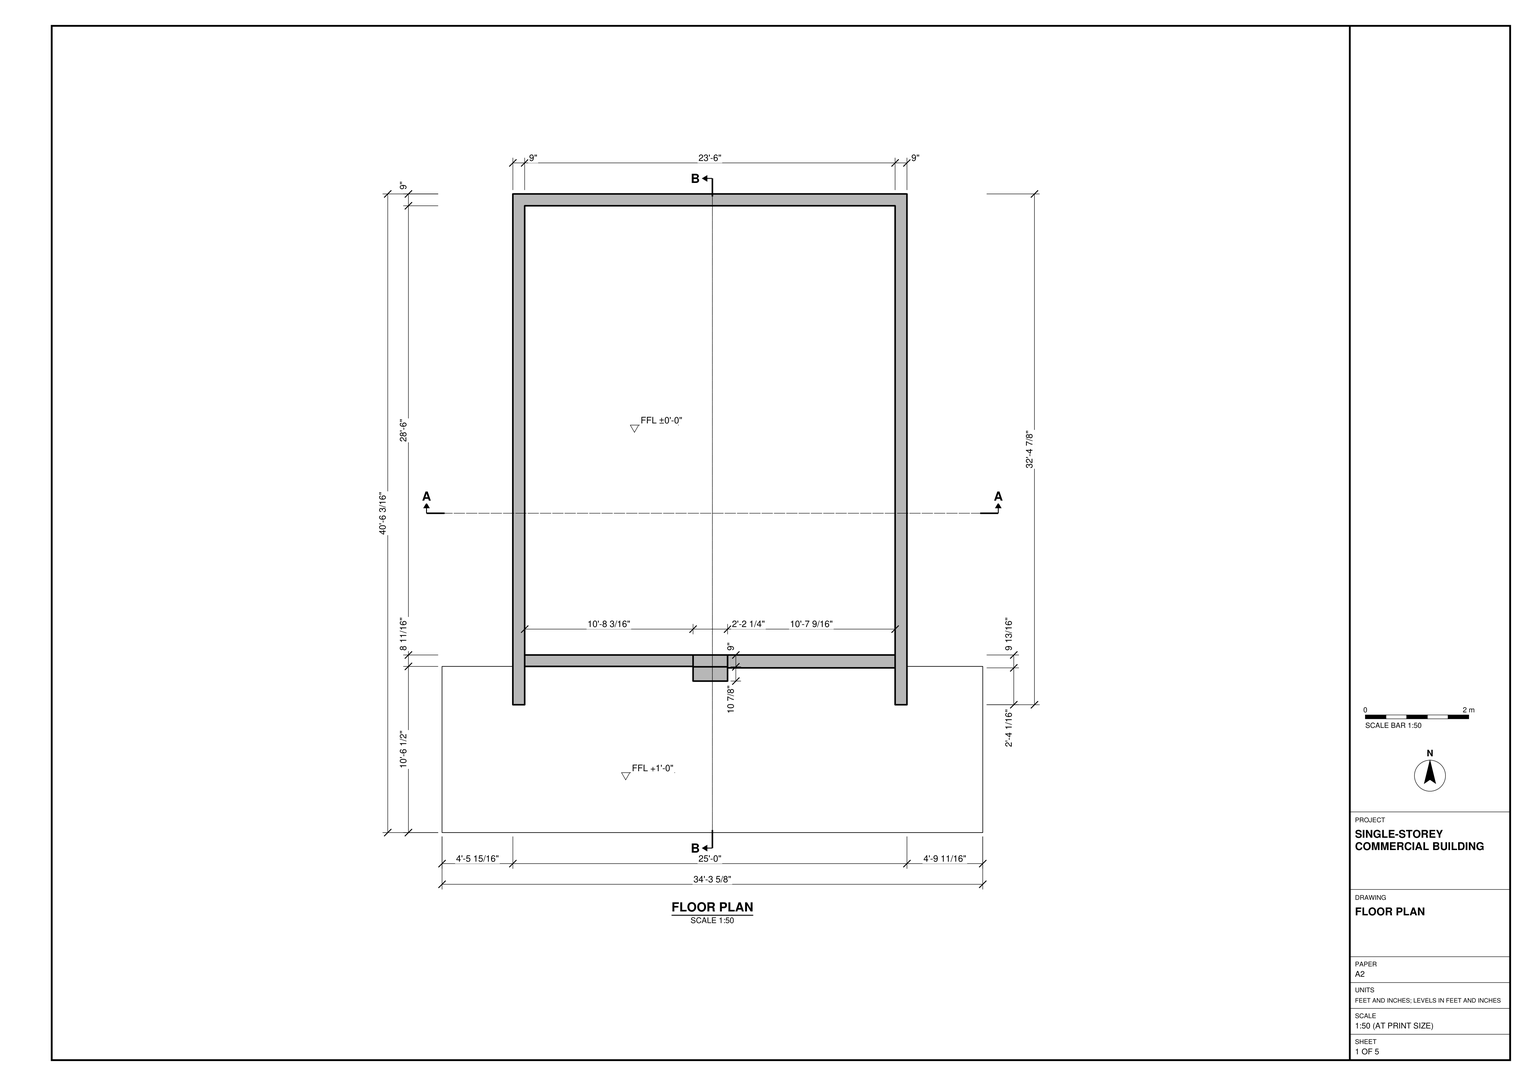
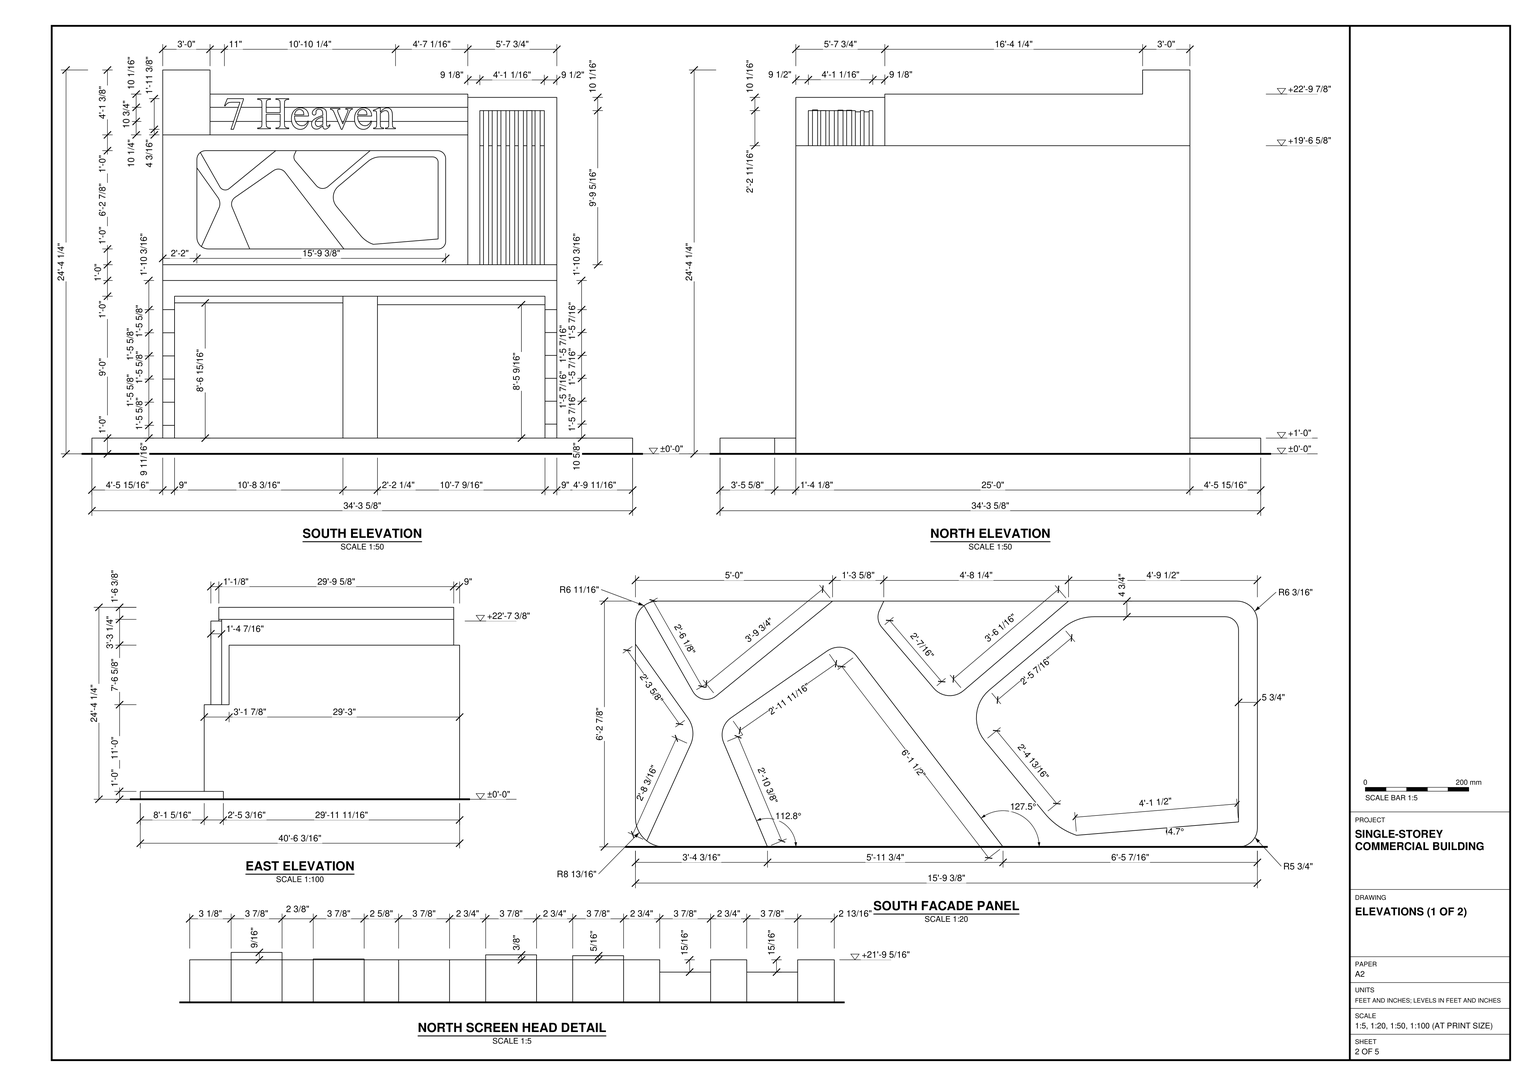
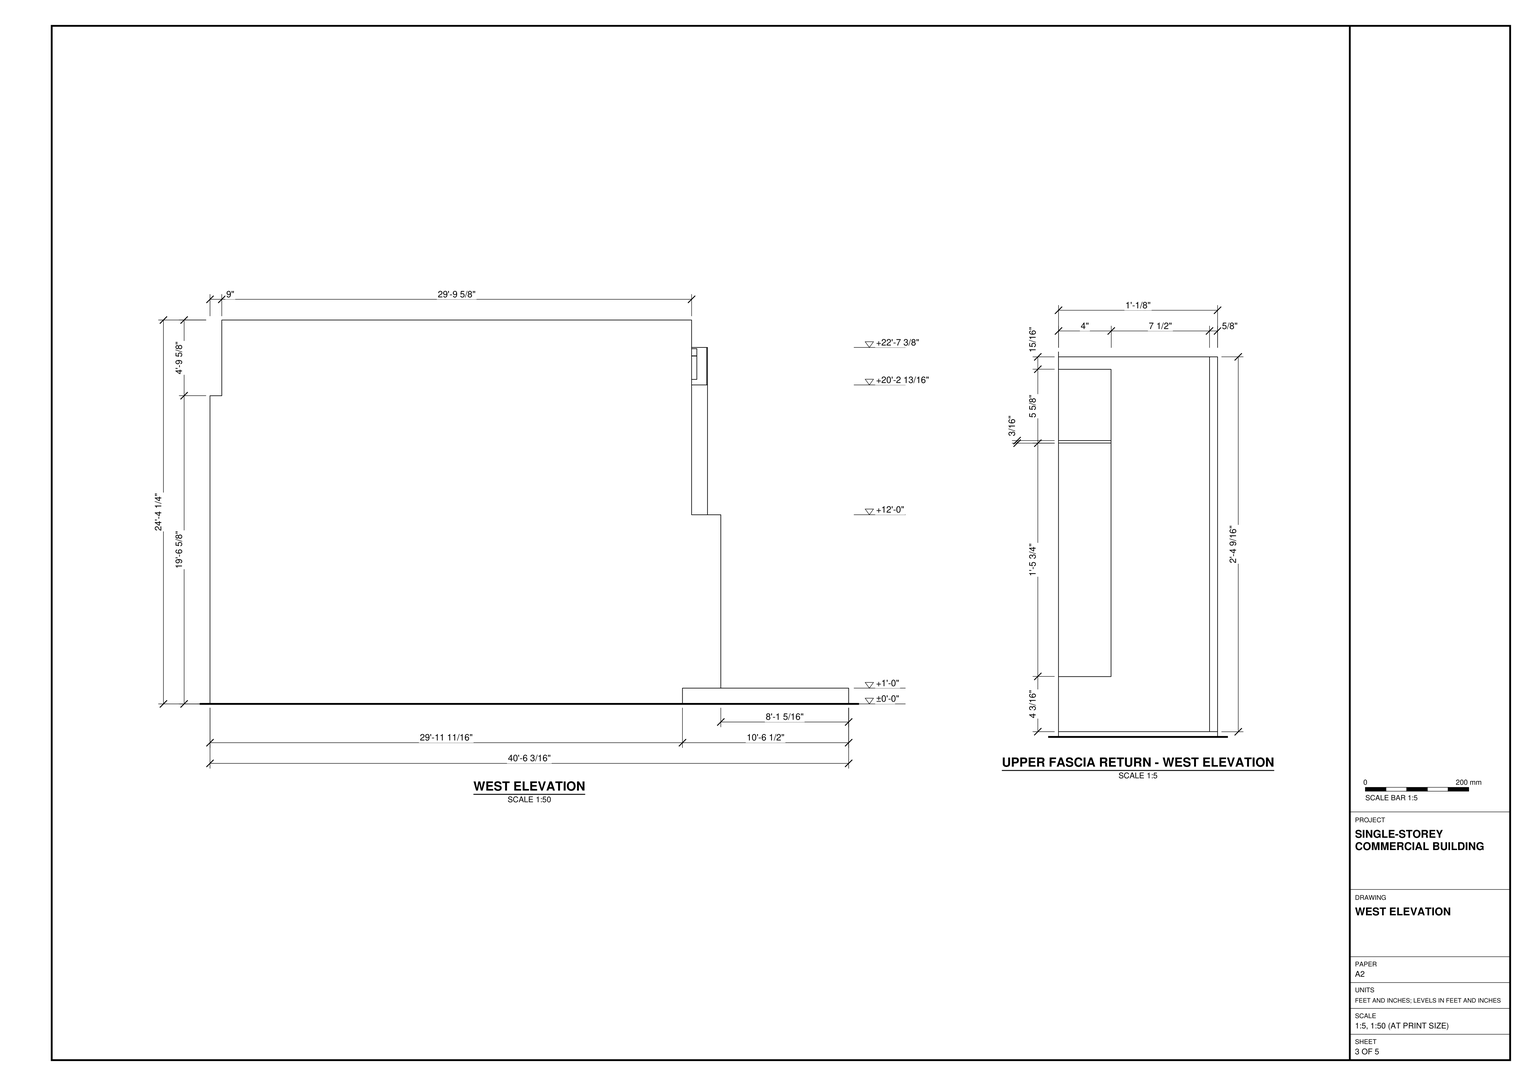
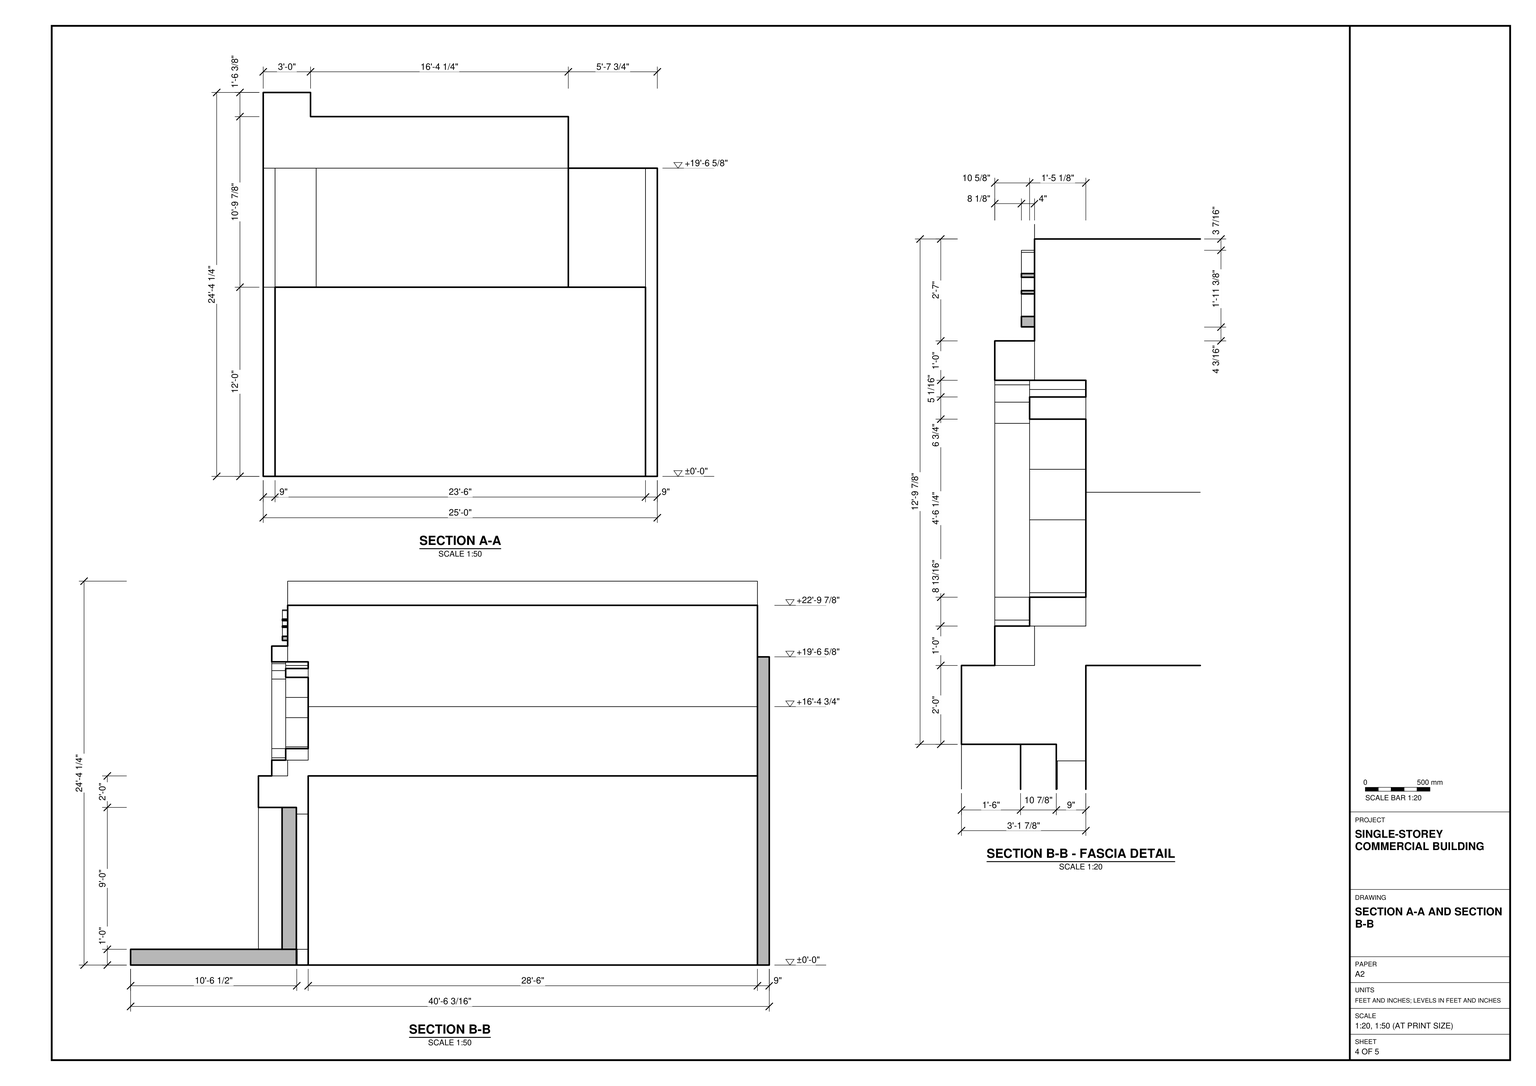
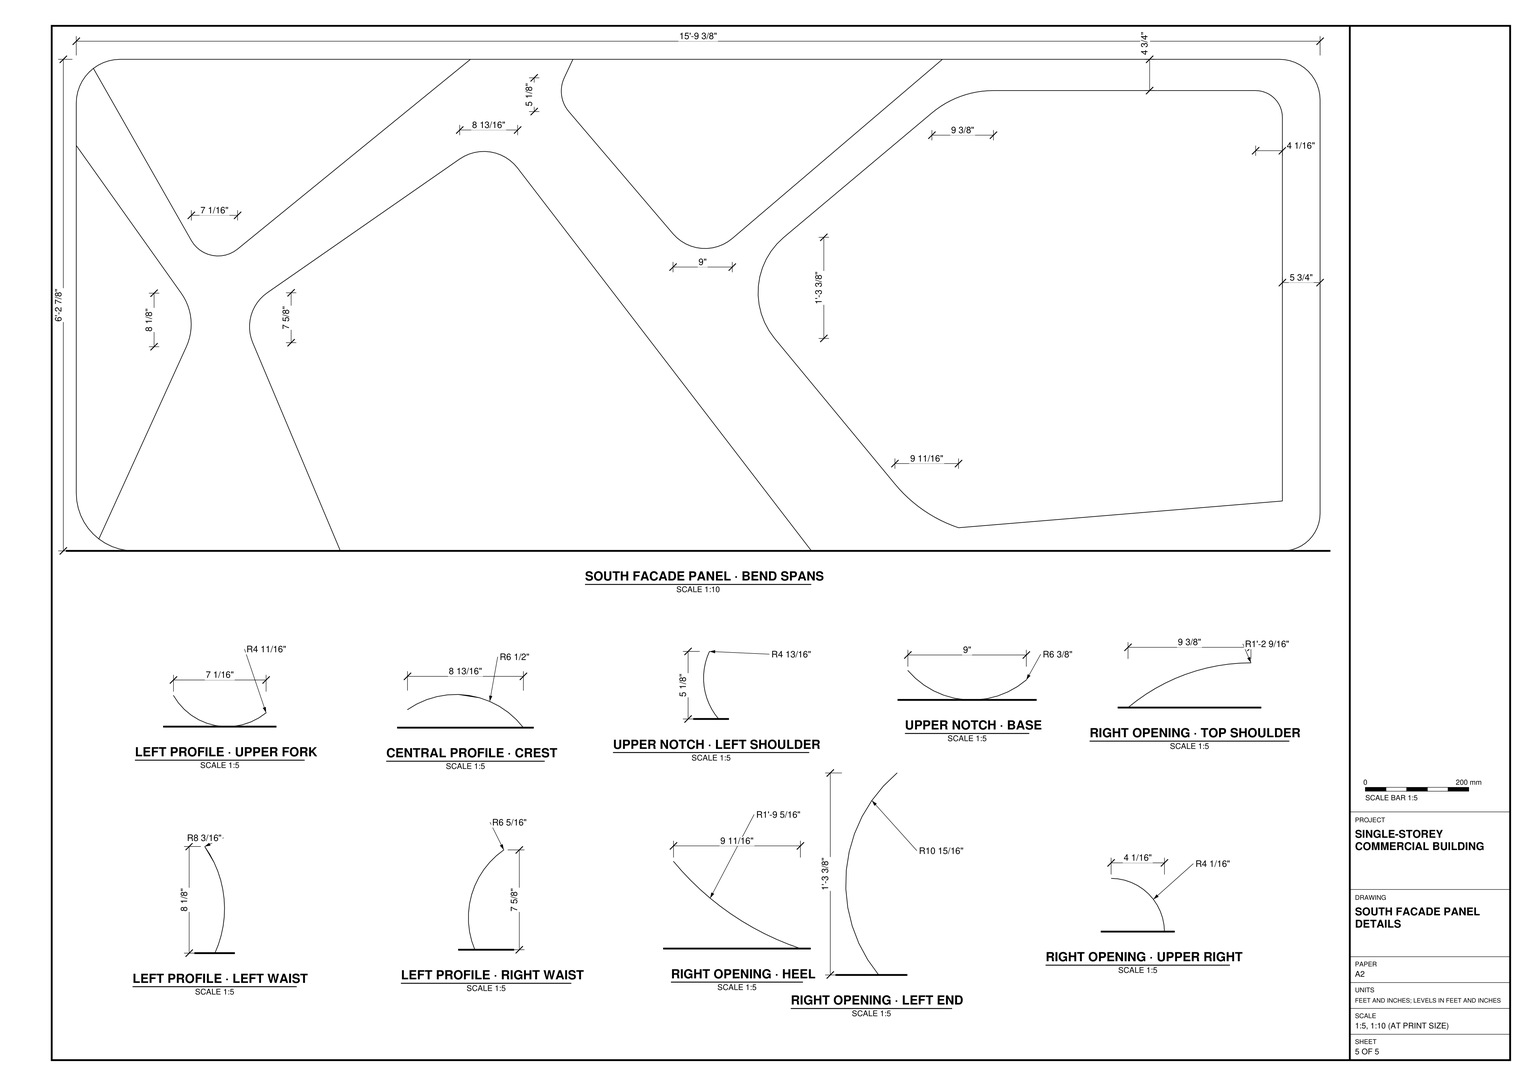
Use task_files/diagram_01.pdf to build the single-storey commercial building in SketchUp. Work in feet and inches. Set the ground-floor datum to ±0'-0". The complete model, including the projecting front platform, measures 34'-3 5/8" east to west, 40'-6 3/16" north to south and 24'-4 1/4" high.

Lay out the rectangular interior using the clear dimensions on the floor plan and the 9" side and rear walls. Extend the side walls past the storefront as drawn. Place the front platform at +1'-0" and follow the plan offsets on each side rather than centring it on the building. Form the two wide storefront bays on either side of the central pier, with a continuous horizontal band above them.

Use the south elevation and its enlarged panel detail to lay out the upper facade. Reproduce the rounded panel outline and branching diagonal pattern, the sign lettering on the horizontal fascia above it, and the narrow vertical screen to its right. Follow the side and rear elevations for the roof, stepped parapet heights and fascia returns.

Keep the walls, slabs, roof and distinct facade elements in separate groups or components, and use components for repeated parts such as screen slats. Any decor or loose items shown may be represented by suitable library components. Save one SketchUp model as output_files/single_storey_commercial_building_with_storefront.skp.

# SketchUp Ruby script. Lengths in inches.
U = 1.inch
M = Sketchup.active_model
def pt(a) = Geom::Point3d.new(a.map { |v| v * U })
def face(e, loops, mat)
  f = e.add_face(loops[0].map { |a| pt(a) })
  loops[1..].each { |l| e.add_face(l.map { |a| pt(a) }).erase! }
  f.material = f.back_material = mat if mat
  f
end
# faces: each face lists its corners as indices into pts; further lists are holes
def faces(e, pts, list, mat = nil) = list.each { |f| face(e, (f[0].is_a?(Array) ? f : [f]).map { |l| l.map { |i| pts[i] } }, mat) }
# xy, xz, yz: faces in a plane at the given z, y or x. An outline is a flat list of corners, or four numbers for a rectangle; further outlines are holes
def ring(l) = l.size == 4 ? [[l[0], l[1]], [l[2], l[1]], [l[2], l[3]], [l[0], l[3]]] : l.each_slice(2).to_a
def flat(e, list, mat, &to3) = list.each { |f| face(e, (f[0].is_a?(Array) ? f : [f]).map { |l| ring(l).map { |u, v| to3.(u, v) } }, mat) }
def xy(e, z, list, mat = nil) = flat(e, list, mat) { |x, y| [x, y, z] }
def xz(e, y, list, mat = nil) = flat(e, list, mat) { |x, z| [x, y, z] }
def yz(e, x, list, mat = nil) = flat(e, list, mat) { |y, z| [x, y, z] }
def lines(e, pts, list) = list.each { |a, b| e.add_line(pt(pts[a]), pt(pts[b])) }
# prism: a flat outline (further loops are holes) pulled along v
def prism(e, loops, v, mat = nil)
  f = face(e, loops, mat); d = Geom::Vector3d.new(v.map { |x| x * U })
  f.pushpull(f.normal.samedirection?(d) ? d.length : -d.length)
end
def box(e, o, s, mat = nil) = prism(e, [[o, [o[0] + s[0], o[1], o[2]], [o[0] + s[0], o[1] + s[1], o[2]], [o[0], o[1] + s[1], o[2]]]], [0, 0, s[2]], mat)
def at(x, y, z, deg = 0) = Geom::Transformation.translation(pt([x, y, z])) * Geom::Transformation.rotation(ORIGIN, Z_AXIS, deg.degrees)
def axes(o, x, y, z) = Geom::Transformation.new([*x, 0, *y, 0, *z, 0, *pt(o).to_a, 1])
def part(name) = M.definitions.add(name)
# library, detail: a bought-in or finely detailed component or shape, given as its bounding box
def library(name, o, s) = part(name).tap { |d| box(d.entities, o, s) }
def detail(e, o, s) = box(e.add_group.entities, o, s)
def put(e, d, t, mat = nil) = e.add_instance(d, t).tap { |i| i.material = mat if mat }
def group(e, t, mat = nil) = e.add_group.tap { |g| g.transformation = t; g.material = mat if mat }.entities
root = M.entities
M.materials.add("[Color B02]").color = [255, 178, 153]
M.materials.add("[Color B03]").color = [255, 140, 101]
M.materials.add("[Color M05]").color = [114, 114, 114]
M.materials.add("[Color M06]").color = [86, 86, 86]
M.materials.add("[Translucent Glass Gray]").color = [128, 128, 128]
M.materials["[Translucent Glass Gray]"].alpha = 0.5
M.materials.add("[Window Covering 02]").color = [199, 178, 115]
c1 = library("7 Heaven\#1",[1.28,0,0],[130.23,23.39,4])
xy(root,0,[[[53.91,126.2,353.91,486.2],[62.91,135.2,344.91,477.2]],[62.91,135.2,344.91,477.2]])
xy(root,12,[[53.91,97.32,62.91,126.2],[344.91,97.32,353.91,126.2],[191.1,115.32,217.37,126.2],[217.37,125.38,344.91,126.2],[62.91,126.2,191.1,126.51],
  [217.37,126.2,344.91,135.2],[62.91,126.51,191.1,135.2]])
xy(root,113.56,[[217.37,125.38,344.91,126.2],[217.37,126.2,344.91,135.2]])
xy(root,114.95,[[62.91,126.2,191.1,126.51],[62.91,126.51,191.1,135.2]])
xy(root,120,[[191.1,115.32,217.37,126.2]])
xy(root,120,[[62.91,97.32,191.1,126.2],[191.1,97.32,217.37,115.32],[217.37,97.32,344.91,126.2]],"[Color B03]")
xy(root,144,[[344.38,107.46,353.91,123.92],[298.1,108.67,301.98,123.92],[304.73,108.67,308.6,123.92],[311.35,108.67,315.23,123.92],[317.98,108.67,321.85,123.92],
  [324.6,108.67,328.48,123.92],[62.91,135.2,286.16,477.2],[286.16,135.2,344.91,477.2]])
xy(root,144,[[[53.91,97.32,353.91,97.32,353.91,107.46,344.38,107.46,344.38,123.92,353.91,123.92,353.91,135.2,286.16,135.2,286.16,123.92,295.3125,123.92,295.3125,107.46,53.91,107.46],[337.35,108.67,341.23,123.92],[331.1,108.67,334.98,123.92],[324.6,108.67,328.48,123.92],[317.98,108.67,321.85,123.92],[311.35,108.67,315.23,123.92],[304.73,108.67,308.6,123.92],[298.1,108.67,301.98,123.92]]],"[Color B03]")
xy(root,156,[[88.7,107.46,120.12,118.07],[120.12,107.46,191.84,135.2],[191.84,107.46,263.57,118.07]],"[Color B02]")
xy(root,226.09,[[219.54,118.07,259.46,135.2]],"[Color B02]")
xy(root,230.84,[[86.58,107.46,139.92,135.2],[139.92,107.46,155.53,118.07],[155.53,107.46,211.78,135.2],[211.78,107.46,263.1,118.07]],"[Color B02]")
xy(root,234.625,[[286.16,135.2,353.91,135.2,353.91,486.2,53.91,486.2,53.91,477.2,286.16,477.2]],"[Color B03]")
xy(root,242.84,[[53.91,107.46,286.16,119.57]],"[Color B02]")
xy(root,261.3125,[[324.6,108.67,328.48,123.92]])
xy(root,261.375,[[331.1,108.67,334.98,123.92]])
xy(root,261.625,[[311.35,108.67,315.23,123.92]])
xy(root,261.6875,[[317.98,108.67,321.85,123.92]])
xy(root,261.875,[[337.35,108.67,341.23,123.92]])
xy(root,271.375,[[286.16,107.46,353.91,123.92]],"[Color M06]")
xy(root,273.875,[[89.91,119.57,286.16,477.2]],"[Color B03]")
xy(root,292.25,[[53.91,119.57,89.91,477.2]],"[Color M05]")
xz(root,97.32,[[53.91,12,62.91,21.69],[344.91,12,353.91,22.63],[53.91,21.69,62.91,39.32],[344.91,22.63,353.91,40.07],[53.91,39.32,62.91,56.94],
  [344.91,40.07,353.91,57.5],[53.91,56.94,62.91,74.57],[344.91,57.5,353.91,74.94],[53.91,74.57,62.91,92.19],[344.91,74.94,353.91,92.38],
  [53.91,92.19,62.91,109.82],[344.91,92.38,353.91,109.82],[53.91,109.82,62.91,109.82,62.91,120,344.91,120,344.91,109.82,353.91,109.82,353.91,132,53.91,132],[53.91,132,353.91,144]],"[Color B03]")
xz(root,107.46,[[[53.91,144,286.16,242.84],[88.7,156,87.55,156.08,86.43,156.3,85.34,156.67,84.31,157.18,83.35,157.82,82.49,158.57,81.73,159.4375,81.09,160.39,80.58,161.43,80.21,162.51,79.99,163.64,79.91,164.79,79.91,224.18,79.97,225.05,80.14,225.9,80.42,226.73,80.8,227.51,81.29,228.24,81.86,228.89,82.52,229.47,83.25,229.95,84.03,230.34,84.85,230.62,85.71,230.79,86.58,230.84,263.1,230.84,263.91,230.79,264.7,230.63,265.47,230.375,266.2,230.02,266.87,229.57,267.48,229.03,268.01,228.43,268.46,227.75,268.82,227.03,269.08,226.26,269.23,225.47,269.29,224.66,269.29,161.72,269.24,160.97,269.09,160.24,268.85,159.53,268.52,158.86,268.1,158.24,267.61,157.68,267.05,157.18,266.43,156.77,265.75,156.4375,265.05,156.19,264.3125,156.05,263.57,156]]],"[Color B02]")
xz(root,107.46,[[286.16,144,295.3125,144,295.3125,261.3125,344.38,261.3125,344.38,144,353.91,144,353.91,271.375,286.16,271.375]],"[Color M06]")
xz(root,108.67,[[298.1,144,301.98,261.3125],[304.73,144,308.6,261.3125],[311.35,144,315.23,261.625],[317.98,144,321.85,261.6875],[324.6,144,328.48,261.3125],
  [331.1,144,334.98,261.375],[337.35,144,341.23,261.875]],"[Color M06]")
xz(root,115.32,[[191.1,12,217.37,120]],"[Color B02]")
xz(root,118.07,[[[88.7,156,120.12,156,106.78,187.7,106.54,188.37,106.38,189.07,106.3,189.77,106.3,190.49,106.38,191.2,106.54,191.89,106.78,192.5625,107.09,193.2,107.47,193.81,107.92,194.36,108.43,194.86,108.99,195.3,138.28,215.66,138.98,216.09,139.73,216.42,140.52,216.65,141.33,216.79,142.15,216.82,142.97,216.74,143.77,216.57,144.54,216.29,145.27,215.92,145.95,215.45,146.56,214.91,147.1,214.29,191.84,156,263.57,156,264.3125,156.05,265.05,156.19,265.75,156.4375,266.43,156.77,267.05,157.18,267.61,157.68,268.1,158.24,268.52,158.86,268.85,159.53,269.09,160.24,269.24,160.97,269.29,161.72,269.29,224.66,269.23,225.47,269.08,226.26,268.82,227.03,268.46,227.75,268.01,228.43,267.48,229.03,266.87,229.57,266.2,230.02,265.47,230.375,264.7,230.63,263.91,230.79,263.1,230.84,211.78,230.84,179.79,203.57,179.12,203.07,178.39,202.66,177.61,202.35,176.8,202.14,175.96,202.05,175.13,202.06,174.3,202.18,173.49,202.41,172.72,202.74,172.01,203.17,171.35,203.6875,170.77,204.29,154.91,222.89,154.625,223.25,154.38,223.64,154.18,224.05,154.01,224.47,153.88,224.91,153.8,225.36,153.76,225.82,153.77,226.28,153.8125,226.73,153.9,227.18,154.04,227.62,154.21,228.04,155.53,230.84,139.92,230.84,104.47,201.96,103.92,201.57,103.31,201.26,102.67,201.05,102,200.93,101.32,200.9,100.64,200.98,99.98,201.15,99.36,201.42,98.78,201.77,98.25,202.21,97.8,202.71,97.42,203.28,82.52,229.47,81.86,228.89,81.29,228.24,80.8,227.51,80.42,226.73,80.14,225.9,79.97,225.05,79.91,224.18,79.91,217.73,95.9,195.22,96.29,194.625,96.62,194,96.9,193.34,97.12,192.66,97.28,191.97,97.375,191.27,97.41,190.55,97.39,189.84,97.3,189.14,97.15,188.44,96.94,187.76,96.68,187.1,83.35,157.82,84.31,157.18,85.34,156.67,86.43,156.3,87.55,156.08],[214.24,159.53,213.3,159.86,212.39,160.24,211.49,160.66,210.62,161.125,209.77,161.63,208.9375,162.17,208.14,162.75,207.36,163.36,206.62,164.01,205.9,164.7,205.22,165.42,204.57,166.16,186.23,188.36,185.39,189.51,184.72,190.77,184.21,192.1,183.875,193.49,183.73,194.91,183.76,196.34,183.98,197.75,184.39,199.11,184.96,200.42,185.7,201.64,186.6,202.75,187.63,203.74,210.18,222.68,210.84,223.2,211.53,223.69,212.26,224.13,213,224.54,213.77,224.9,214.56,225.21,215.36,225.48,216.18,225.69,217.01,225.87,217.85,225.99,218.6875,226.0625,219.54,226.09,259.46,226.09,260,226.05,260.52,225.95,261.03,225.78,261.51,225.54,261.95,225.24,262.35,224.89,262.7,224.49,263,224.04,263.24,223.57,263.41,223.06,263.51,222.54,263.55,222,263.55,163.6]]],"[Color B02]")
xz(root,119.57,[[89.91,242.84,286.16,253.07],[89.91,253.07,286.16,263.82],[89.91,263.82,286.16,273.875]],"[Color B03]")
xz(root,119.57,[[53.91,242.84,89.91,292.25]],"[Color M05]")
xz(root,123.92,[[311.35,261.3125,315.23,261.625],[317.98,261.3125,321.85,261.6875],[331.1,261.3125,334.98,261.375]])
xz(root,123.92,[[286.16,144,286.16,271.375,353.91,271.375,353.91,144,344.38,144,344.38,261.3125,341.23,261.3125,341.23,261.875,337.35,261.875,337.35,261.3125,334.98,261.3125,334.98,261.375,331.1,261.375,331.1,261.3125,321.85,261.3125,321.85,261.6875,317.98,261.6875,317.98,261.3125,315.23,261.3125,315.23,261.625,311.35,261.625,311.35,261.3125,308.6,261.3125,308.6,260.375,304.73,260.375,304.73,261.3125,301.98,261.3125,301.98,260.375,298.1,260.375,298.1,261.3125,295.3125,261.3125,295.3125,144],[298.1,144,301.98,260.375],[304.73,144,308.6,260.375],[311.35,144,315.23,261.3125],[317.98,144,321.85,261.3125],
  [324.6,144,328.48,261.3125],[331.1,144,334.98,261.3125],[337.35,144,341.23,261.3125],[337.35,261.3125,341.23,261.875]],"[Color M06]")
xz(root,125.38,[[217.37,12,344.91,113.56]],"[Window Covering 02]")
xz(root,126.2,[[53.91,0,353.91,12],[191.1,12,217.37,120]])
xz(root,126.2,[[217.37,113.56,344.91,120],[62.91,114.95,191.1,120]],"[Color B03]")
xz(root,126.51,[[62.91,12,191.1,114.95]],"[Window Covering 02]")
xz(root,135.2,[[62.91,0,62.91,12,191.1,12,191.1,114.95,62.91,114.95,62.91,144,344.91,144,344.91,113.56,217.37,113.56,217.37,12,344.91,12,344.91,0],[62.91,12,191.1,114.95],[217.37,12,344.91,113.56]])
xz(root,135.2,[[286.16,144,344.91,234.625],[344.91,144,353.91,234.625]],"[Color B03]")
xz(root,135.2,[[120.12,156,191.84,156,147.1,214.29,146.56,214.91,145.95,215.45,145.27,215.92,144.54,216.29,143.77,216.57,142.97,216.74,142.15,216.82,141.33,216.79,140.52,216.65,139.73,216.42,138.98,216.09,138.28,215.66,108.99,195.3,108.43,194.86,107.92,194.36,107.47,193.81,107.09,193.2,106.78,192.5625,106.54,191.89,106.38,191.2,106.3,190.49,106.3,189.77,106.38,189.07,106.54,188.37,106.78,187.7],[83.35,157.82,96.68,187.1,96.94,187.76,97.15,188.44,97.3,189.14,97.39,189.84,97.41,190.55,97.375,191.27,97.28,191.97,97.12,192.66,96.9,193.34,96.62,194,96.29,194.625,95.9,195.22,79.91,217.73,79.91,164.79,79.99,163.64,80.21,162.51,80.58,161.43,81.09,160.39,81.73,159.4375,82.49,158.57],[214.24,159.53,263.55,163.6,263.55,222,263.51,222.54,263.41,223.06,263.24,223.57,263,224.04,262.7,224.49,262.35,224.89,261.95,225.24,261.51,225.54,261.03,225.78,260.52,225.95,260,226.05,259.46,226.09,219.54,226.09,218.6875,226.0625,217.85,225.99,217.01,225.87,216.18,225.69,215.36,225.48,214.56,225.21,213.77,224.9,213,224.54,212.26,224.13,211.53,223.69,210.84,223.2,210.18,222.68,187.63,203.74,186.6,202.75,185.7,201.64,184.96,200.42,184.39,199.11,183.98,197.75,183.76,196.34,183.73,194.91,183.875,193.49,184.21,192.1,184.72,190.77,185.39,189.51,186.23,188.36,204.57,166.16,205.22,165.42,205.9,164.7,206.62,164.01,207.36,163.36,208.14,162.75,208.9375,162.17,209.77,161.63,210.62,161.125,211.49,160.66,212.39,160.24,213.3,159.86],[101.32,200.9,102,200.93,102.67,201.05,103.31,201.26,103.92,201.57,104.47,201.96,139.92,230.84,86.58,230.84,85.71,230.79,84.85,230.62,84.03,230.34,83.25,229.95,82.52,229.47,97.42,203.28,97.8,202.71,98.25,202.21,98.78,201.77,99.36,201.42,99.98,201.15,100.64,200.98],[175.96,202.05,176.8,202.14,177.61,202.35,178.39,202.66,179.12,203.07,179.79,203.57,211.78,230.84,155.53,230.84,154.21,228.04,154.04,227.62,153.9,227.18,153.8125,226.73,153.77,226.28,153.76,225.82,153.8,225.36,153.88,224.91,154.01,224.47,154.18,224.05,154.38,223.64,154.625,223.25,154.91,222.89,170.77,204.29,171.35,203.6875,172.01,203.17,172.72,202.74,173.49,202.41,174.3,202.18,175.13,202.06]],"[Translucent Glass Gray]")
xz(root,477.2,[[62.91,0,344.91,144],[62.91,144,94.22,234.625],[94.22,144,286.16,234.625]])
xz(root,477.2,[[53.91,234.625,53.91,292.25,89.91,292.25,89.91,273.875,286.16,273.875,286.16,234.625]],"[Color B03]")
xz(root,486.2,[[53.91,0,353.91,234.625]],"[Color B03]")
yz(root,53.91,[[107.46,144,119.57,242.84]],"[Color B02]")
yz(root,53.91,[[126.2,0,126.2,12,97.32,12,97.32,144,119.57,144,119.57,292.25,477.2,292.25,477.2,234.625,486.2,234.625,486.2,0]],"[Color B03]")
yz(root,62.91,[[135.2,0,477.2,144],[126.51,12,135.2,114.95]])
yz(root,62.91,[[97.32,12,126.51,12,126.51,114.95,126.2,114.95,126.2,120,97.32,120]],"[Color B03]")
yz(root,79.91,[[107.46,164.79,135.2,217.73],[107.46,217.73,118.07,224.18]],"[Color B02]")
yz(root,89.91,[[119.57,273.875,477.2,292.25]],"[Color M05]")
yz(root,106.3,[[118.07,189.77,135.2,190.49]],"[Color B02]")
yz(root,191.1,[[126.2,12,126.51,114.95],[126.51,12,135.2,114.95]])
yz(root,191.1,[[115.32,12,126.2,120]],"[Color B02]")
yz(root,217.37,[[125.38,12,126.2,113.56],[126.2,12,135.2,113.56]])
yz(root,217.37,[[115.32,12,125.38,12,125.38,113.56,126.2,113.56,126.2,120,115.32,120]],"[Color B02]")
yz(root,263.55,[[118.07,163.6,135.2,222]],"[Color B02]")
yz(root,269.29,[[107.46,161.72,118.07,224.66]],"[Color B02]")
yz(root,286.16,[[107.46,144,123.92,144,123.92,271.375,119.57,271.375,119.57,242.84,107.46,242.84],[135.2,144,477.2,234.625]])
yz(root,286.16,[[123.92,144,135.2,144,135.2,234.625,477.2,234.625,477.2,273.875,123.92,273.875],[119.57,271.375,123.92,273.875]],"[Color B03]")
yz(root,286.16,[[107.46,242.84,108.07,271.375],[108.07,242.84,119.57,271.375]],"[Color M06]")
yz(root,295.3125,[[107.46,144,123.92,261.3125]],"[Color M06]")
yz(root,298.1,[[108.67,144,123.92,261.3125]],"[Color M06]")
yz(root,301.98,[[108.67,144,123.92,261.3125]],"[Color M06]")
yz(root,304.73,[[108.67,144,123.92,261.3125]],"[Color M06]")
yz(root,308.6,[[108.67,144,123.92,261.3125]],"[Color M06]")
yz(root,311.35,[[108.67,144,123.92,261.625]],"[Color M06]")
yz(root,315.23,[[108.67,144,123.92,261.625]],"[Color M06]")
yz(root,317.98,[[108.67,144,123.92,261.6875]],"[Color M06]")
yz(root,321.85,[[108.67,144,123.92,261.6875]],"[Color M06]")
yz(root,324.6,[[108.67,144,123.92,261.3125]],"[Color M06]")
yz(root,328.48,[[108.67,144,123.92,261.3125]],"[Color M06]")
yz(root,331.1,[[108.67,144,123.92,261.375]],"[Color M06]")
yz(root,334.98,[[108.67,144,123.92,261.375]],"[Color M06]")
yz(root,337.35,[[108.67,144,123.92,261.875]],"[Color M06]")
yz(root,341.23,[[108.67,144,123.92,261.875]],"[Color M06]")
yz(root,344.38,[[107.46,144,123.92,261.3125]],"[Color M06]")
yz(root,344.91,[[135.2,0,477.2,144],[125.38,12,135.2,113.56]])
yz(root,344.91,[[97.32,12,97.32,120,126.2,120,126.2,113.56,125.38,113.56,125.38,12]],"[Color B03]")
yz(root,353.91,[[126.2,0,486.2,0,486.2,234.625,135.2,234.625,135.2,144,97.32,144,97.32,12,126.2,12]],"[Color B03]")
yz(root,353.91,[[107.46,144,123.92,271.375]],"[Color M06]")
p = [[88.7,107.46,156],[88.7,118.07,156],[87.55,118.07,156.08],[87.55,107.46,156.08],[264.3125,107.46,156.05],[264.3125,118.07,156.05],
  [263.57,118.07,156],[263.57,107.46,156],[265.05,107.46,156.19],[265.05,118.07,156.19],[120.12,135.2,156],[106.78,135.2,187.7],
  [106.78,118.07,187.7],[120.12,118.07,156],[147.1,135.2,214.29],[191.84,135.2,156],[191.84,118.07,156],[147.1,118.07,214.29],
  [86.43,118.07,156.3],[86.43,107.46,156.3],[265.75,107.46,156.4375],[265.75,118.07,156.4375],[85.34,118.07,156.67],[85.34,107.46,156.67],
  [266.43,107.46,156.77],[266.43,118.07,156.77],[84.31,118.07,157.18],[84.31,107.46,157.18],[267.05,107.46,157.18],[267.05,118.07,157.18],
  [83.35,118.07,157.82],[83.35,107.46,157.82],[267.61,107.46,157.68],[267.61,118.07,157.68],[268.1,107.46,158.24],[268.1,118.07,158.24],
  [83.35,135.2,157.82],[82.49,135.2,158.57],[82.49,107.46,158.57],[96.68,135.2,187.1],[96.68,118.07,187.1],[268.52,107.46,158.86],
  [268.52,118.07,158.86],[81.73,135.2,159.4375],[81.73,107.46,159.4375],[268.85,107.46,159.53],[268.85,118.07,159.53],[81.09,135.2,160.39],
  [81.09,107.46,160.39],[269.09,107.46,160.24],[269.09,118.07,160.24],[214.24,135.2,159.53],[213.3,135.2,159.86],[213.3,118.07,159.86],
  [214.24,118.07,159.53],[263.55,135.2,163.6],[263.55,118.07,163.6],[212.39,135.2,160.24],[212.39,118.07,160.24],[269.24,107.46,160.97],
  [269.24,118.07,160.97],[211.49,135.2,160.66],[211.49,118.07,160.66],[80.58,135.2,161.43],[80.58,107.46,161.43],[210.62,135.2,161.125],
  [210.62,118.07,161.125],[269.29,107.46,161.72],[269.29,118.07,161.72],[209.77,135.2,161.63],[209.77,118.07,161.63],[80.21,135.2,162.51],
  [80.21,107.46,162.51],[208.9375,135.2,162.17],[208.9375,118.07,162.17],[208.14,135.2,162.75],[208.14,118.07,162.75],[79.99,135.2,163.64],
  [79.99,107.46,163.64],[207.36,135.2,163.36],[207.36,118.07,163.36],[206.62,135.2,164.01],[206.62,118.07,164.01],[79.91,135.2,164.79],
  [79.91,107.46,164.79],[205.9,135.2,164.7],[205.9,118.07,164.7],[205.22,135.2,165.42],[205.22,118.07,165.42],[204.57,135.2,166.16],
  [204.57,118.07,166.16],[186.23,135.2,188.36],[186.23,118.07,188.36],[96.94,135.2,187.76],[96.94,118.07,187.76],[106.54,135.2,188.37],
  [106.54,118.07,188.37],[97.15,135.2,188.44],[97.15,118.07,188.44],[97.3,135.2,189.14],[97.3,118.07,189.14],[106.38,135.2,189.07],
  [106.38,118.07,189.07],[185.39,135.2,189.51],[185.39,118.07,189.51],[97.39,135.2,189.84],[97.39,118.07,189.84],[106.3,135.2,189.77],
  [106.3,118.07,189.77],[184.72,135.2,190.77],[184.72,118.07,190.77],[97.41,135.2,190.55],[97.41,118.07,190.55],[106.3,135.2,190.49],
  [106.38,135.2,191.2],[106.38,118.07,191.2],[106.3,118.07,190.49],[97.375,135.2,191.27],[97.375,118.07,191.27],[184.21,135.2,192.1],
  [184.21,118.07,192.1],[106.54,135.2,191.89],[106.54,118.07,191.89],[97.28,135.2,191.97],[97.28,118.07,191.97],[106.78,135.2,192.5625],
  [106.78,118.07,192.5625],[97.12,135.2,192.66],[97.12,118.07,192.66],[183.875,135.2,193.49],[183.875,118.07,193.49],[107.09,135.2,193.2],
  [107.09,118.07,193.2],[96.9,135.2,193.34],[96.9,118.07,193.34],[107.47,135.2,193.81],[107.47,118.07,193.81],[96.62,135.2,194],
  [96.62,118.07,194],[183.73,135.2,194.91],[183.73,118.07,194.91],[107.92,135.2,194.36],[107.92,118.07,194.36],[96.29,135.2,194.625],
  [96.29,118.07,194.625],[108.43,135.2,194.86],[108.43,118.07,194.86],[95.9,135.2,195.22],[95.9,118.07,195.22],[108.99,135.2,195.3],
  [108.99,118.07,195.3],[183.76,135.2,196.34],[183.76,118.07,196.34],[79.91,135.2,217.73],[79.91,118.07,217.73],[138.28,135.2,215.66],
  [138.28,118.07,215.66],[183.98,135.2,197.75],[183.98,118.07,197.75],[184.39,135.2,199.11],[184.39,118.07,199.11],[184.96,135.2,200.42],
  [184.96,118.07,200.42],[185.7,135.2,201.64],[185.7,118.07,201.64],[101.32,135.2,200.9],[100.64,135.2,200.98],[100.64,118.07,200.98],
  [101.32,118.07,200.9],[102,135.2,200.93],[102,118.07,200.93],[102.67,135.2,201.05],[102.67,118.07,201.05],[99.98,135.2,201.15],
  [99.98,118.07,201.15],[103.31,135.2,201.26],[103.31,118.07,201.26],[99.36,135.2,201.42],[99.36,118.07,201.42],[103.92,135.2,201.57],
  [103.92,118.07,201.57],[98.78,135.2,201.77],[98.78,118.07,201.77],[104.47,135.2,201.96],[104.47,118.07,201.96],[186.6,135.2,202.75],
  [186.6,118.07,202.75],[98.25,135.2,202.21],[98.25,118.07,202.21],[139.92,135.2,230.84],[139.92,118.07,230.84],[175.96,135.2,202.05],
  [175.13,135.2,202.06],[175.13,118.07,202.06],[175.96,118.07,202.05],[176.8,135.2,202.14],[176.8,118.07,202.14],[174.3,135.2,202.18],
  [174.3,118.07,202.18],[177.61,135.2,202.35],[177.61,118.07,202.35],[97.8,135.2,202.71],[97.8,118.07,202.71],[173.49,135.2,202.41],
  [173.49,118.07,202.41],[178.39,135.2,202.66],[178.39,118.07,202.66],[172.72,135.2,202.74],[172.72,118.07,202.74],[97.42,135.2,203.28],
  [97.42,118.07,203.28],[172.01,135.2,203.17],[172.01,118.07,203.17],[179.12,135.2,203.07],[179.12,118.07,203.07],[187.63,135.2,203.74],
  [187.63,118.07,203.74],[179.79,135.2,203.57],[179.79,118.07,203.57],[171.35,135.2,203.6875],[171.35,118.07,203.6875],[82.52,135.2,229.47],
  [82.52,118.07,229.47],[211.78,135.2,230.84],[211.78,118.07,230.84],[170.77,135.2,204.29],[170.77,118.07,204.29],[210.18,135.2,222.68],
  [210.18,118.07,222.68],[154.91,135.2,222.89],[154.91,118.07,222.89],[146.56,135.2,214.91],[146.56,118.07,214.91],[145.95,135.2,215.45],
  [145.95,118.07,215.45],[145.27,135.2,215.92],[145.27,118.07,215.92],[138.98,135.2,216.09],[138.98,118.07,216.09],[144.54,135.2,216.29],
  [144.54,118.07,216.29],[139.73,135.2,216.42],[139.73,118.07,216.42],[143.77,135.2,216.57],[143.77,118.07,216.57],[140.52,135.2,216.65],
  [140.52,118.07,216.65],[142.97,135.2,216.74],[142.97,118.07,216.74],[141.33,135.2,216.79],[141.33,118.07,216.79],[142.15,135.2,216.82],
  [142.15,118.07,216.82],[263.51,135.2,222.54],[263.55,135.2,222],[263.55,118.07,222],[263.51,118.07,222.54],[263.41,135.2,223.06],
  [263.41,118.07,223.06],[210.84,135.2,223.2],[210.84,118.07,223.2],[154.625,135.2,223.25],[154.625,118.07,223.25],[263.24,135.2,223.57],
  [263.24,118.07,223.57],[154.38,135.2,223.64],[154.38,118.07,223.64],[211.53,135.2,223.69],[211.53,118.07,223.69],[154.18,135.2,224.05],
  [154.18,118.07,224.05],[263,135.2,224.04],[263,118.07,224.04],[212.26,135.2,224.13],[212.26,118.07,224.13],[154.01,135.2,224.47],
  [154.01,118.07,224.47],[262.7,135.2,224.49],[262.7,118.07,224.49],[213,135.2,224.54],[213,118.07,224.54],[79.91,107.46,224.18],
  [79.91,118.07,224.18],[79.97,118.07,225.05],[79.97,107.46,225.05],[153.88,135.2,224.91],[153.88,118.07,224.91],[213.77,135.2,224.9],
  [213.77,118.07,224.9],[262.35,135.2,224.89],[262.35,118.07,224.89],[269.23,107.46,225.47],[269.23,118.07,225.47],[269.29,118.07,224.66],
  [269.29,107.46,224.66],[153.8,135.2,225.36],[153.8,118.07,225.36],[214.56,135.2,225.21],[214.56,118.07,225.21],[261.95,135.2,225.24],
  [261.95,118.07,225.24],[80.14,118.07,225.9],[80.14,107.46,225.9],[215.36,135.2,225.48],[215.36,118.07,225.48],[261.51,135.2,225.54],
  [261.51,118.07,225.54],[153.76,135.2,225.82],[153.76,118.07,225.82],[269.08,107.46,226.26],[269.08,118.07,226.26],[216.18,135.2,225.69],
  [216.18,118.07,225.69],[261.03,135.2,225.78],[261.03,118.07,225.78],[217.01,135.2,225.87],[217.01,118.07,225.87],[153.77,135.2,226.28],
  [153.77,118.07,226.28],[260.52,135.2,225.95],[260.52,118.07,225.95],[80.42,118.07,226.73],[80.42,107.46,226.73],[217.85,135.2,225.99],
  [217.85,118.07,225.99],[260,135.2,226.05],[260,118.07,226.05],[218.6875,135.2,226.0625],[218.6875,118.07,226.0625],[219.54,135.2,226.09],
  [219.54,118.07,226.09],[259.46,135.2,226.09],[259.46,118.07,226.09],[268.82,107.46,227.03],[268.82,118.07,227.03],[153.8125,135.2,226.73],
  [153.8125,118.07,226.73],[80.8,118.07,227.51],[80.8,107.46,227.51],[153.9,135.2,227.18],[153.9,118.07,227.18],[268.46,107.46,227.75],
  [268.46,118.07,227.75],[154.04,135.2,227.62],[154.04,118.07,227.62],[81.29,118.07,228.24],[81.29,107.46,228.24],[154.21,135.2,228.04],
  [154.21,118.07,228.04],[268.01,107.46,228.43],[268.01,118.07,228.43],[155.53,135.2,230.84],[155.53,118.07,230.84],[81.86,118.07,228.89],
  [81.86,107.46,228.89],[267.48,107.46,229.03],[267.48,118.07,229.03],[82.52,107.46,229.47],[266.87,107.46,229.57],[266.87,118.07,229.57],
  [83.25,135.2,229.95],[83.25,107.46,229.95],[266.2,107.46,230.02],[266.2,118.07,230.02],[84.03,135.2,230.34],[84.03,107.46,230.34],
  [265.47,107.46,230.375],[265.47,118.07,230.375],[84.85,135.2,230.62],[84.85,107.46,230.62],[264.7,107.46,230.63],[264.7,118.07,230.63],
  [85.71,135.2,230.79],[85.71,107.46,230.79],[263.91,107.46,230.79],[263.91,118.07,230.79],[86.58,135.2,230.84],[86.58,107.46,230.84],
  [263.1,107.46,230.84],[263.1,118.07,230.84],[353.91,126.2,120],[344.91,126.2,120],[62.91,126.2,120],[53.91,126.2,120],
  [179.3,135.2,196.74],[179.3,481.38,196.74],[62.91,477.2,144],[53.91,477.2,144],[344.91,477.2,144],[344.91,477.2,234.625]]
faces(root,p,[[0,1,2,3],[4,5,6,7],[8,9,5,4],[10,11,12,13],[14,15,16,17],[3,2,18,19],[20,21,9,8],[19,18,22,23],
  [24,25,21,20],[23,22,26,27],[28,29,25,24],[27,26,30,31],[32,33,29,28],[34,35,33,32],[36,37,38,31,30],[39,36,30,40],
  [41,42,35,34],[37,43,44,38],[45,46,42,41],[43,47,48,44],[49,50,46,45],[51,52,53,54],[55,51,54,56],[52,57,58,53],
  [59,60,50,49],[57,61,62,58],[47,63,64,48],[61,65,66,62],[67,68,60,59],[65,69,70,66],[63,71,72,64],[69,73,74,70],
  [73,75,76,74],[71,77,78,72],[75,79,80,76],[79,81,82,80],[77,83,84,78],[81,85,86,82],[85,87,88,86],[87,89,90,88],
  [89,91,92,90],[93,39,40,94],[11,95,96,12],[97,93,94,98],[99,97,98,100],[95,101,102,96],[91,103,104,92],[105,99,100,106],
  [101,107,108,102],[103,109,110,104],[111,105,106,112],[113,114,115,116],[117,111,112,118],[109,119,120,110],[114,121,122,115],[123,117,118,124],
  [121,125,126,122],[127,123,124,128],[119,129,130,120],[125,131,132,126],[133,127,128,134],[131,135,136,132],[137,133,134,138],[129,139,140,130],
  [135,141,142,136],[143,137,138,144],[141,145,146,142],[147,143,144,148],[145,149,150,146],[139,151,152,140],[153,147,148,154],[149,155,156,150],
  [151,157,158,152],[157,159,160,158],[159,161,162,160],[161,163,164,162],[165,166,167,168],[169,165,168,170],[171,169,170,172],[166,173,174,167],
  [175,171,172,176],[173,177,178,174],[179,175,176,180],[177,181,182,178],[183,179,180,184],[163,185,186,164],[181,187,188,182],[189,183,184,190],
  [191,192,193,194],[195,191,194,196],[192,197,198,193],[199,195,196,200],[187,201,202,188],[197,203,204,198],[205,199,200,206],[203,207,208,204],
  [201,209,210,202],[207,211,212,208],[213,205,206,214],[185,215,216,186],[217,213,214,218],[211,219,220,212],[209,221,222,210],[223,217,218,224],
  [219,225,226,220],[215,227,228,216],[225,229,230,226],[231,14,17,232],[233,231,232,234],[235,233,234,236],[155,237,238,156],[239,235,236,240],
  [237,241,242,238],[243,239,240,244],[241,245,246,242],[247,243,244,248],[245,249,250,246],[251,247,248,252],[249,251,252,250],[253,254,255,256],
  [257,253,256,258],[227,259,260,228],[229,261,262,230],[263,257,258,264],[261,265,266,262],[259,267,268,260],[265,269,270,266],[271,263,264,272],
  [267,273,274,268],[269,275,276,270],[277,271,272,278],[273,279,280,274],[281,282,283,284],[275,285,286,276],[279,287,288,280],[289,277,278,290],
  [291,292,293,294],[285,295,296,286],[287,297,298,288],[299,289,290,300],[284,283,301,302],[297,303,304,298],[305,299,300,306],[295,307,308,296],
  [309,310,292,291],[303,311,312,304],[313,305,306,314],[311,315,316,312],[307,317,318,308],[319,313,314,320],[302,301,321,322],[315,323,324,316],
  [325,319,320,326],[323,327,328,324],[327,329,330,328],[331,325,326,332],[333,334,310,309],[317,335,336,318],[322,321,337,338],[335,339,340,336],
  [341,342,334,333],[339,343,344,340],[338,337,345,346],[343,347,348,344],[349,350,342,341],[347,351,352,348],[346,345,353,354],[355,356,350,349],
  [354,353,222,357],[358,359,356,355],[221,360,361,357,222],[362,363,359,358],[360,364,365,361],[366,367,363,362],[364,368,369,365],[370,371,367,366],
  [368,372,373,369],[374,375,371,370],[372,376,377,373],[378,379,375,374]],"[Color B02]")
lines(root,p,[[380,381],[382,383],[384,385],[386,387],[388,389]])
put(root,c1,axes([99.6,119.57,247.03],[1,0,0],[0,0,1],[0,-1,0]))
g1 = group(root,at(0,0,0),"[Color B02]")
prism(g1,[[[370.03,126.5,0],[411.625,126.5,0],[411.625,0,0],[0,0,0],[0,126.5,0],[70.03,126.5,0],[207.22,126.5,0],[233.49,126.5,0]]],[0,0,12])
